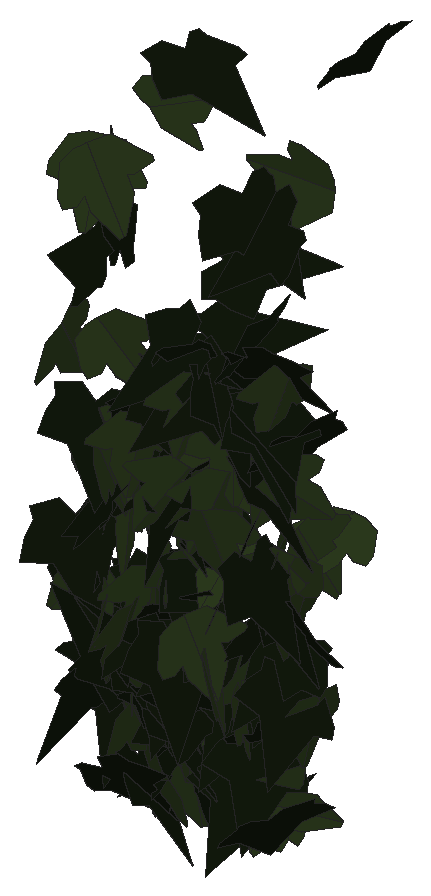
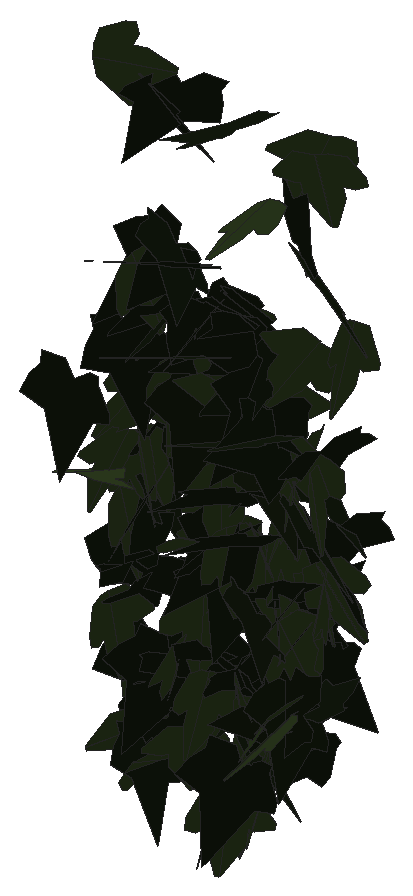
# SketchUp Ruby script. Lengths in inches.
U = 1.inch
M = Sketchup.active_model
def pt(a) = Geom::Point3d.new(a.map { |v| v * U })
def face(e, loops, mat)
  f = e.add_face(loops[0].map { |a| pt(a) })
  loops[1..].each { |l| e.add_face(l.map { |a| pt(a) }).erase! }
  f.material = f.back_material = mat if mat
  f
end
# faces: each face lists its corners as indices into pts; further lists are holes
def faces(e, pts, list, mat = nil) = list.each { |f| face(e, (f[0].is_a?(Array) ? f : [f]).map { |l| l.map { |i| pts[i] } }, mat) }
# xy, xz, yz: faces in a plane at the given z, y or x. An outline is a flat list of corners, or four numbers for a rectangle; further outlines are holes
def ring(l) = l.size == 4 ? [[l[0], l[1]], [l[2], l[1]], [l[2], l[3]], [l[0], l[3]]] : l.each_slice(2).to_a
def flat(e, list, mat, &to3) = list.each { |f| face(e, (f[0].is_a?(Array) ? f : [f]).map { |l| ring(l).map { |u, v| to3.(u, v) } }, mat) }
def xy(e, z, list, mat = nil) = flat(e, list, mat) { |x, y| [x, y, z] }
def xz(e, y, list, mat = nil) = flat(e, list, mat) { |x, z| [x, y, z] }
def yz(e, x, list, mat = nil) = flat(e, list, mat) { |y, z| [x, y, z] }
def lines(e, pts, list) = list.each { |a, b| e.add_line(pt(pts[a]), pt(pts[b])) }
# prism: a flat outline (further loops are holes) pulled along v
def prism(e, loops, v, mat = nil)
  f = face(e, loops, mat); d = Geom::Vector3d.new(v.map { |x| x * U })
  f.pushpull(f.normal.samedirection?(d) ? d.length : -d.length)
end
def box(e, o, s, mat = nil) = prism(e, [[o, [o[0] + s[0], o[1], o[2]], [o[0] + s[0], o[1] + s[1], o[2]], [o[0], o[1] + s[1], o[2]]]], [0, 0, s[2]], mat)
def at(x, y, z, deg = 0) = Geom::Transformation.translation(pt([x, y, z])) * Geom::Transformation.rotation(ORIGIN, Z_AXIS, deg.degrees)
def axes(o, x, y, z) = Geom::Transformation.new([*x, 0, *y, 0, *z, 0, *pt(o).to_a, 1])
def part(name) = M.definitions.add(name)
# library, detail: a bought-in or finely detailed component or shape, given as its bounding box
def library(name, o, s) = part(name).tap { |d| box(d.entities, o, s) }
def detail(e, o, s) = box(e.add_group.entities, o, s)
def put(e, d, t, mat = nil) = e.add_instance(d, t).tap { |i| i.material = mat if mat }
def group(e, t, mat = nil) = e.add_group.tap { |g| g.transformation = t; g.material = mat if mat }.entities
root = M.entities
M.materials.add("efeu1").color = [18, 25, 13]
M.materials.add("efeu2").color = [43, 57, 29]
c1 = part("ivyleaf_10")
p = [[0,0.5,-0.03],[-0.0625,2.02,-0.43],[-0.19,2.01,-0.46],[-0.54,1.05,-0.29],[-0.52,0.625,-0.18],[-0.83,0.76,-0.28],
  [-1.16,0.64,-0.33],[-1.15,0.33,-0.24],[-0.77,-0.39,0.02],[-0.3,-0.51,0.16],[0.04,-0.48,0.23],[-0.02,2.01,-0.4375],
  [-0.06,2.01,-0.43],[0.04,-0.49,0.23],[0.67,-0.49,0.14],[1.38,0.36,-0.2],[1.375,0.51,-0.24],[0.81,0.65,-0.19],
  [0.62,0.59,-0.15],[0.6,1.09,-0.28],[0.5,1.23,-0.31]]
faces(c1.entities,p,[[0,1,2,3,4,5,6,7,8,9,10],[11,12,0,13,14,15,16,17,18,19,20]],"efeu2")
c2 = part("ivyleaf_9")
p = [[1.54,2.16,1.25],[1.36,2.04,1.19],[-0.21,0.99,0.68],[-0.71,1.11,0.82],[-0.85,0.86,0.67],[-0.8,0.17,0.21],
  [-0.9,-0.01,0.1],[-0.67,-0.16,-0.02],[-0.08,-0.08,-0.05],[-0.03,-0.6,-0.4],[0.65,-0.88,-0.66],[0.83,-0.6,-0.49],
  [1.29,-0.42,-0.43],[1.8125,-0.07,-0.26],[1.21,0.44,0.15]]
faces(c2.entities,p,[[0,1,2,3,4,5,6,7,8,9,10,11,12,13,14]],"efeu1")
put(root,c1,axes([591.4375,126.52,287.95],[0.46801,-1.07376,0.00249],[0.12711,0.05271,-1.16321],[1.06621,0.46504,0.13758]))
put(root,c2,axes([591.24,125.21,283.37],[-0.61835,0.80711,0.73771],[0.37892,-0.63682,1.01434],[1.02571,0.72183,0.07001]))
put(root,c1,axes([591.59,124.4375,292.5625],[0.01609,-1.06662,-0.66344],[0.13317,0.66121,-1.0598],[1.24904,-0.05676,0.12154]))
put(root,c1,axes([592.01,125.15,283.89],[0.94792,0.02402,-0.71315],[-0.70038,0.25815,-0.92225],[0.1365,1.1578,0.22042]))
put(root,c2,axes([592.48,125.31,295.13],[-0.74096,0.82574,0.5679],[-0.38395,0.41848,-1.10943],[-0.92571,-0.83451,0.00559]))
put(root,c1,axes([591.29,128.47,279.91],[0.72194,-0.73393,-0.64288],[0.58744,0.96551,-0.44257],[0.77902,-0.0479,0.92951]))
put(root,c2,axes([592.33,126.41,286.8],[-0.95137,0.70352,-0.09598],[0.08355,-0.04843,-1.18319],[-0.7051,-0.95497,-0.0107]))
put(root,c2,axes([592.16,126.74,279.72],[0.06356,1.15918,0.3041],[0.00135,0.30446,-1.16083],[-1.1984,0.06183,0.01482]))
put(root,c1,axes([591.36,126.12,283.94],[0.60877,-0.84993,0.577],[0.68424,-0.1648,-0.96466],[0.76624,0.82242,0.40301]))
put(root,c2,axes([591.54,126.04,289.16],[-0.14595,-1.18109,-0.17242],[0.06089,0.16611,-1.18941],[1.19205,-0.15309,0.03964]))
put(root,c2,axes([592.33,138.08,296.75],[0.11446,1.17684,0.20971],[-0.03269,0.21367,-1.18123],[-1.19494,0.10688,0.05241]))
put(root,c2,axes([591.49,126.85,279.67],[-0.26854,-0.97066,0.57114],[0.6311,-0.616,-0.75016],[0.93278,0.13733,0.67197]))
put(root,c2,axes([591.75,124.84,285.72],[-0.2533,-1.02103,-0.58523],[0.13503,0.56946,-1.05197],[1.16909,-0.287,-0.00529]))
put(root,c2,axes([592.29,125.17,280.34],[-0.31245,0.53168,-1.01304],[0.41286,-0.92699,-0.61385],[-1.067,-0.51438,0.05914]))
put(root,c1,axes([592.15,128.5625,298.94],[1.08326,-0.28479,-0.55372],[0.26313,1.2164,-0.11086],[0.56433,-0.0205,1.11457]))
put(root,c2,axes([592.31,126.96,279.07],[-0.41702,-1.09053,0.07911],[0.01919,-0.09196,-1.16644],[1.09323,-0.41438,0.05066]))
put(root,c2,axes([591.59,127.18,279.79],[0.95242,-0.36758,0.55902],[0.59218,0.01058,-1.00196],[0.31135,1.1043,0.19567]))
put(root,c1,axes([592.74,126.37,281.95],[-0.31205,-1.025,0.45467],[-0.06424,-0.45483,-1.06945],[1.11948,-0.31181,0.06537]))
put(root,c1,axes([591.95,128.34,279.85],[-0.22771,-1.023,0.53845],[0.91714,-0.49395,-0.55061],[0.70379,0.31271,0.89175]))
put(root,c1,axes([592,125.91,288.57],[0.98692,0.29131,0.68503],[0.6591,0.1868,-1.029],[-0.34601,1.18676,-0.00618]))
put(root,c1,axes([592.52,124.93,298.98],[1.1722,0.4523,-0.07607],[-0.0607,-0.05395,-1.25611],[-0.45462,1.17343,-0.02843]))
put(root,c2,axes([593.42,124.41,287.08],[-0.75565,0.88999,0.03043],[-0.15188,-0.08948,-1.15453],[-0.87746,-0.75095,0.17363]))
put(root,c1,axes([592.97,124.47,283.39],[0.78719,-0.88646,-0.20753],[-0.11645,0.17406,-1.1852],[0.90295,0.79527,0.02807]))
put(root,c1,axes([592.875,124.85,288.45],[-0.40582,1.06458,0.32695],[-0.10769,0.30883,-1.13927],[-1.10844,-0.41977,-0.00901]))
put(root,c2,axes([593.25,125.11,295.97],[0.41127,-0.28071,1.15398],[-0.33976,1.14236,0.39898],[-1.13799,-0.44252,0.29793]))
put(root,c1,axes([592.97,126.3,286.84],[-0.84999,0.81382,0.03331],[-0.01951,0.02779,-1.17675],[-0.81427,-0.85019,-0.00658]))
put(root,c1,axes([592.47,125.5,292.26],[0.83062,0.45329,0.72541],[0.46288,0.61211,-0.91251],[-0.71933,0.91732,0.25045]))
put(root,c2,axes([593.59,126.96,282.74],[-0.14977,0.88899,0.74331],[-0.29087,0.69665,-0.8918],[-1.1217,-0.29935,0.13201]))
put(root,c1,axes([593.04,125,281.42],[-1.08464,0.48857,-0.04164],[0.03868,-0.01551,-1.1896],[-0.48882,-1.08533,-0.00174]))
put(root,c2,axes([593.15,126.71,289.33],[-0.36282,0.7987,-0.78771],[-0.32394,0.71802,0.87725],[1.074,0.48638,-0.00151]))
put(root,c2,axes([593.87,126.05,287.26],[-0.29539,1.05041,0.51491],[-0.45123,0.38767,-1.04969],[-1.0793,-0.44956,0.29793]))
put(root,c2,axes([592.66,127.01,282.87],[0.43663,-1.07671,0.08982],[0.04849,-0.07725,-1.16176],[1.07936,0.43902,0.01586]))
put(root,c2,axes([593.86,124.81,281.1875],[0.41101,-0.01919,1.19464],[-1.17972,0.19356,0.40899],[-0.18922,-1.24845,0.04505]))
put(root,c2,axes([593.28,128.18,277.61],[0.64234,0.97487,-0.01908],[-0.00678,-0.01839,-1.16745],[-0.97503,0.64236,-0.00445]))
put(root,c2,axes([592.35,128.25,290.17],[0.75,-0.92775,-0.38454],[0.61174,0.80266,-0.74337],[0.79647,0.25713,0.93307]))
put(root,c1,axes([593.08,125.72,286.54],[1.0293,-0.54814,0.29844],[0.29971,-0.07079,-1.16368],[0.54745,1.06935,0.07594]))
put(root,c2,axes([593.88,125.51,281.08],[-0.02828,-0.04278,1.25851],[-0.18442,1.24539,0.03819],[-1.24566,-0.18341,-0.03422]))
put(root,c1,axes([593,124.16,299.18],[0.72923,0.93638,0.44496],[0.30336,0.32747,-1.1863],[-0.99134,0.789,-0.0357]))
put(root,c1,axes([593.33,127.31,275.96],[-0.72216,0.89475,-0.19022],[0.11369,-0.15268,-1.1498],[-0.90766,-0.73102,0.00732]))
put(root,c1,axes([593.44,125.59,279.16],[0.00754,-0.99563,-0.59524],[0.18606,0.58859,-0.98213],[1.14497,-0.08909,0.16352]))
put(root,c2,axes([593.19,124.54,277.42],[1.09712,0.40483,0.1263],[0.11535,0.05221,-1.1694],[-0.40808,1.10314,0.009]))
put(root,c2,axes([593.15,126.05,280.9],[0.53483,-1.02385,-0.13399],[-0.05333,0.1233,-1.15508],[1.0312,0.53739,0.00975]))
put(root,c1,axes([593.8,128.15,276.05],[-0.8752,-0.75615,-0.11022],[0.08791,0.06683,-1.15658],[0.75906,-0.87957,0.00687]))
put(root,c1,axes([593.82,124.68,283],[0.17237,-1.18206,0.10636],[-0.00777,-0.1086,-1.19434],[1.18681,0.17097,-0.02327]))
put(root,c2,axes([593.55,125.83,290.3],[0.85155,0.8684,0.2679],[0.17211,0.20639,-1.21607],[-0.89234,0.86852,0.02111]))
put(root,c2,axes([593.87,126.42,283.26],[-0.81605,-0.84941,0.16483],[0.05952,-0.28115,-1.15413],[0.8632,-0.78362,0.23541]))
put(root,c2,axes([594.42,126.46,277.79],[-0.90614,0.71886,-0.01641],[0.00982,-0.01402,-1.15665],[-0.71898,-0.90618,0.00488]))
put(root,c2,axes([593.29,126.125,277.1],[0.80795,-0.93243,-0.22441],[-0.14518,0.17114,-1.23378],[0.948,0.82089,0.00232]))
put(root,c2,axes([593.02,128.26,286.41],[0.50495,-0.88763,-0.6331],[0.52979,0.80955,-0.71247],[0.9529,0.02027,0.73161]))
put(root,c1,axes([594.46,125.81,276.96],[-0.94005,0.31079,0.73922],[-0.70104,0.23453,-0.99009],[-0.38934,-1.17266,-0.0021]))
put(root,c1,axes([594.02,125.2,289.64],[-0.60339,-1.02735,0.23072],[0.05479,-0.29619,-1.17559],[1.05151,-0.57409,0.19365]))
put(root,c1,axes([594.03,126.7,278.6],[-1.04281,0.49449,-0.00391],[0.0035,-0.00174,-1.15412],[-0.4945,-1.04282,0.00007]))
put(root,c1,axes([594.17,125.62,284.09],[-0.59023,-1.06919,0.12767],[0.02657,-0.16001,-1.21719],[1.07646,-0.5823,0.10005]))
put(root,c2,axes([594.49,127.44,276.92],[0.54279,-0.12279,-1.03457],[-0.92821,0.47276,-0.5431],[0.47311,1.06839,0.12142]))
put(root,c2,axes([594.2,127.09,280.58],[-0.40017,-1.08531,0.1492],[-0.009,-0.15558,-1.15586],[1.09548,-0.39774,0.04501]))
put(root,c1,axes([594.0625,127.12,279.67],[0.83529,-0.71026,0.39583],[0.35566,-0.19116,-1.09353],[0.7312,0.90435,0.07972]))
put(root,c2,axes([593.49,128.25,301.5],[0.53515,-1.12245,-0.21247],[0.56634,0.46444,-1.02712],[0.99212,0.34033,0.70093]))
put(root,c1,axes([593.82,126.17,284.04],[-0.10524,-0.10752,-1.16255],[0.6642,-0.96548,0.02917],[-0.96017,-0.65609,0.14759]))
put(root,c2,axes([593.66,128.06,287.76],[0.50433,-0.83811,-0.7007],[0.52918,0.8626,-0.65088],[0.9557,-0.03535,0.73016]))
put(root,c2,axes([593.89,126.16,291.15],[1.00572,-0.61192,0.16135],[0.14957,-0.06454,-1.17704],[0.6149,1.01654,0.0224]))
put(root,c2,axes([594.99,125.56,280.31],[0.56404,0.74499,-0.75413],[-0.48474,-0.57843,-0.93398],[-0.94273,0.74315,0.02904]))
put(root,c2,axes([594.13,125.98,287.59],[0.71634,-0.94,-0.05223],[-0.01024,0.05784,-1.18153],[0.94139,0.71591,0.02689]))
put(root,c1,axes([594.97,126.61,284.65],[-0.32275,-1.13811,0.01923],[0.00789,-0.02223,-1.18291],[1.13825,-0.32256,0.01366]))
put(root,c2,axes([595.61,126.11,279.71],[-1.04776,0.3785,0.34047],[-0.32735,0.09577,-1.11385],[-0.3899,-1.09752,0.02022]))
put(root,c2,axes([594.1875,126.35,279.14],[0.58718,-0.98945,0.09964],[0.21052,0.01059,-1.13547],[0.97192,0.59548,0.18575]))
put(root,c2,axes([595.07,125.65,283.45],[0.65395,0.96259,-0.06883],[-0.16749,0.03132,-1.15323],[-0.9504,0.65682,0.15588]))
put(root,c2,axes([595.79,125.38,293.08],[-1.1856,0.12473,0.03765],[-0.04328,-0.05197,-1.19082],[-0.12289,-1.18506,0.05619]))
put(root,c1,axes([595.78,124.93,288.57],[-0.65048,-0.7406,0.69449],[-0.46066,-0.51972,-0.9857],[0.90476,-0.79707,-0.00257]))
put(root,c1,axes([595.51,126.35,286.79],[-0.75448,-0.92194,-0.00246],[0.09961,-0.07835,-1.18455],[0.91655,-0.7504,0.12671]))
put(root,c1,axes([595.44,127.22,279.42],[-0.336,-0.99066,-0.48377],[0.18672,0.4473,-1.04566],[1.08654,-0.38322,0.03009]))
put(root,c2,axes([594.99,126.34,284.89],[1.16202,0.28427,-0.00735],[-0.00758,0.00005,-1.19628],[-0.28426,1.16204,0.00185]))
put(root,c2,axes([595.4375,125.15,288.35],[-0.95727,0.09461,-0.72432],[0.72386,-0.03746,-0.96155],[-0.09808,-1.19983,-0.0271]))
put(root,c2,axes([595.29,126.56,284.53],[0.20464,-1.08175,-0.44392],[0.02606,0.45477,-1.09618],[1.169,0.17923,0.10215]))
put(root,c2,axes([595.05,127.57,292.12],[1.13393,-0.24621,-0.35657],[0.15269,1.16187,-0.31672],[0.40552,0.251,1.11629]))
put(root,c2,axes([595.06,125.06,291.55],[0.42854,-0.09339,-1.18657],[0.37842,1.20639,0.04172],[1.12848,-0.36908,0.43661]))
put(root,c2,axes([596.55,125.79,292.6875],[0.09563,0.71603,-0.96847],[-0.55141,-0.8377,-0.67379],[-1.07078,0.49532,0.26048]))
put(root,c1,axes([595.96,127.55,284.87],[-1.08514,-0.27303,0.33641],[0.18366,-1.11157,-0.30971],[0.39241,-0.23475,1.07524]))
put(root,c2,axes([595.57,125.02,282.39],[-0.00461,-1.26429,-0.03826],[0.00229,0.03825,-1.2643],[1.26487,-0.00467,0.00215]))
put(root,c1,axes([595.78,127.62,277.72],[0.77203,0.84344,-0.02459],[-0.00214,-0.03138,-1.14326],[-0.8438,0.77179,-0.0196]))
put(root,c2,axes([596.67,125.85,283.09],[-1.15795,-0.21931,0.1775],[-0.17956,-0.00554,-1.17821],[0.21763,-1.17146,-0.02766]))
put(root,c1,axes([596.32,125.26,291.8],[-0.42469,-1.13415,0.37068],[-0.01408,-0.38867,-1.20532],[1.19311,-0.40829,0.11772]))
put(root,c1,axes([596.41,126.25,281.68],[-0.99353,-0.60302,0.01928],[-0.02081,-0.00288,-1.16219],[0.60297,-0.99371,-0.00834]))
put(root,c2,axes([596.89,125.28,292.14],[-1.20583,-0.1099,0.15137],[-0.15186,-0.00146,-1.21077],[0.10923,-1.2153,-0.01223]))
put(root,c2,axes([596.57,125.97,289.18],[0.25469,1.17838,0.31632],[-0.00143,0.32343,-1.2037],[-1.22009,0.24561,0.06744]))
put(root,c1,axes([596.84,125.64,288.32],[-0.43658,-1.01558,0.47968],[-0.08544,-0.48313,-1.10063],[1.11991,-0.43276,0.10303]))
put(root,c2,axes([595.76,127.4,295.25],[1.05103,-0.43487,-0.45442],[0.33162,1.13507,-0.31924],[0.53445,0.15091,1.09172]))
put(root,c2,axes([596.89,127.19,280.17],[-0.85959,-0.77741,-0.01579],[0.01692,0.00483,-1.15896],[0.77739,-0.85972,0.00777]))
put(root,c1,axes([596.43,125.74,289.36],[0.67409,0.78266,0.71109],[0.31977,0.65293,-1.02178],[-1.00795,0.73057,0.1514]))
put(root,c1,axes([596.78,124.27,283.63],[0.60328,0.97589,0.42223],[0.09922,0.43168,-1.13948],[-1.05868,0.59656,0.13382]))
put(root,c1,axes([596.99,126.72,280.2],[-0.28331,1.18421,-0.03155],[0.00831,-0.03045,-1.21762],[-1.1846,-0.28343,-0.00099]))
put(root,c1,axes([597.2,125.9,290.1],[-0.93571,-0.76233,0.03479],[0.12668,-0.20945,-1.18237],[0.75254,-0.91263,0.24229]))
put(root,c2,axes([597.27,126.82,277.49],[-0.7221,-0.9,0.04438],[-0.02741,-0.0349,-1.15388],[0.90068,-0.72262,0.00046]))
put(root,c1,axes([597.26,124.63,287.61],[-1.17452,-0.34539,-0.19391],[0.17324,0.09777,-1.22345],[0.35621,-1.1864,-0.04437]))
put(root,c1,axes([597.33,124.53,282.39],[-0.63491,1.00602,0.25695],[-0.1883,0.18462,-1.18814],[-1.0211,-0.65958,0.05933]))
put(root,c2,axes([596.85,125.73,291.83],[0.44337,-1.13121,0.01637],[0.00131,-0.01707,-1.21499],[1.13133,0.44334,-0.00501]))
put(root,c2,axes([597.9375,127.25,276.41],[-0.27869,1.11691,0.13877],[-0.00117,0.14267,-1.15067],[-1.12549,-0.27671,-0.03316]))
put(root,c1,axes([597.38,128.08,276.32],[-0.71094,-0.42947,0.77584],[0.37781,-1.04632,-0.23298],[0.80226,0.11216,0.79724]))
put(root,c2,axes([597.64,126.48,279.39],[0.67503,0.94644,0.089],[0.04328,0.07844,-1.16246],[-0.94963,0.67634,0.01028]))
put(root,c2,axes([597.76,126.81,278.69],[-0.4645,-1.06379,-0.0732],[0.03386,0.06509,-1.16077],[1.06577,-0.4657,0.00497]))
put(root,c2,axes([598.43,125.09,294.01],[-0.09791,1.03475,0.63578],[-0.24271,0.6083,-1.02741],[-1.18996,-0.20921,0.15725]))
put(root,c2,axes([598.27,125.35,287.26],[-0.69974,0.44726,-0.83712],[0.66709,-0.50805,-0.82905],[-0.67513,-0.96555,0.04846]))
put(root,c2,axes([599.13,125.17,284.7],[-0.84577,0.82767,-0.03501],[0.02093,-0.02868,-1.18336],[-0.82815,-0.84601,0.00586]))
put(root,c2,axes([598.84,127.03,282.79],[-0.90661,-0.72803,0.12405],[-0.04696,-0.13918,-1.16008],[0.73703,-0.90441,0.07867]))
put(root,c1,axes([598.12,126.43,277.04],[0.28676,0.23435,1.15344],[0.5613,1.01626,-0.34602],[-1.03454,0.61634,0.13197]))
put(root,c1,axes([598.83,126.17,286.58],[0.56159,-1.05252,-0.11899],[0.00628,0.13799,-1.1909],[1.0592,0.55723,0.07015]))
put(root,c2,axes([598.24,125.61,289.19],[0.80583,-0.90449,0.13717],[0.15788,-0.04255,-1.20811],[0.90111,0.81631,0.08901]))
put(root,c1,axes([599.51,125.74,286.3],[-0.78339,-0.75221,0.50739],[-0.35474,-0.36306,-1.08596],[0.83512,-0.85984,0.01466]))
put(root,c2,axes([598.41,125.79,291.44],[0.43142,-1.11758,0.19461],[0.20062,-0.12976,-1.18991],[1.11652,0.45515,0.13861]))
put(root,c2,axes([598.66,124.61,299.71],[-0.12594,-0.77016,-1.0234],[0.20637,1.0027,-0.77997],[1.26408,-0.24043,0.02537]))
put(root,c1,axes([599.27,126.59,284.67],[0.06746,-1.22382,-0.02856],[-0.04085,0.02633,-1.22505],[1.22347,0.06836,-0.03933]))
put(root,c2,axes([598.66,124.99,293.76],[1.16958,0.32562,0.09535],[0.06988,0.10374,-1.21136],[-0.33202,1.16887,0.08095]))
put(root,c2,axes([598.79,125.83,285.13],[0.69003,-0.8234,-0.47872],[-0.32162,0.35499,-1.07417],[0.8965,0.76111,-0.0169]))
put(root,c2,axes([598.625,127.03,283.27],[1.24016,-0.40697,-0.16293],[0.15657,-0.04543,1.30522],[-0.40946,-1.25,0.00561]))
put(root,c2,axes([599.56,126.05,290.8125],[0.00977,1.16074,-0.31388],[-0.00817,-0.31382,-1.16077],[-1.2024,0.01156,0.00533]))
put(root,c1,axes([599.44,125.68,293],[-0.23465,-1.13394,0.36765],[0.00227,-0.37513,-1.15556],[1.19205,-0.2225,0.07457]))
put(root,c1,axes([598.98,125.92,289.08],[-0.46803,-0.69567,-0.84847],[0.61253,0.59965,-0.82954],[0.91031,-0.76116,0.12194]))
put(root,c2,axes([598.95,125.59,291.77],[-0.01118,-1.15401,-0.32636],[0.02841,0.32602,-1.15381],[1.19893,-0.01849,0.0243]))
put(root,c2,axes([599.24,126.42,281.45],[-0.3514,-1.1043,0.19735],[0.04113,-0.21935,-1.15416],[1.12104,-0.33811,0.10421]))
put(root,c1,axes([599.58,126.92,280.85],[-0.13724,-1.1541,0.02566],[0.01238,-0.02731,-1.16213],[1.15432,-0.13692,0.01552]))
put(root,c1,axes([599.56,128.4375,286.55],[-1.16974,-0.07396,0.07872],[0.0634,-1.16327,-0.15078],[0.08744,-0.14589,1.16234]))
put(root,c2,axes([599.2,124.375,286.88],[0.39078,-0.9301,-0.68902],[-0.27329,0.63253,-1.00885],[1.12479,0.47683,-0.00573]))
put(root,c2,axes([600.22,124.65,299.21],[-1.2066,0.19295,-0.0226],[0.02183,-0.0066,-1.22193],[-0.19304,-1.2068,0.00307]))
put(root,c2,axes([600.03,124.16,278.16],[0.2616,1.25673,-0.14425],[-0.22561,-0.09859,-1.26807],[-1.2447,0.282,0.19952]))
put(root,c1,axes([599.58,126.61,286.85],[0.05217,1.04428,0.55607],[-0.05002,0.55806,-1.04332],[-1.18204,0.02247,0.0687]))
put(root,c1,axes([600.6875,125.57,300.47],[-0.05641,-0.0053,-1.21676],[-1.21032,0.12553,0.05557],[0.12515,1.21159,-0.01108]))
